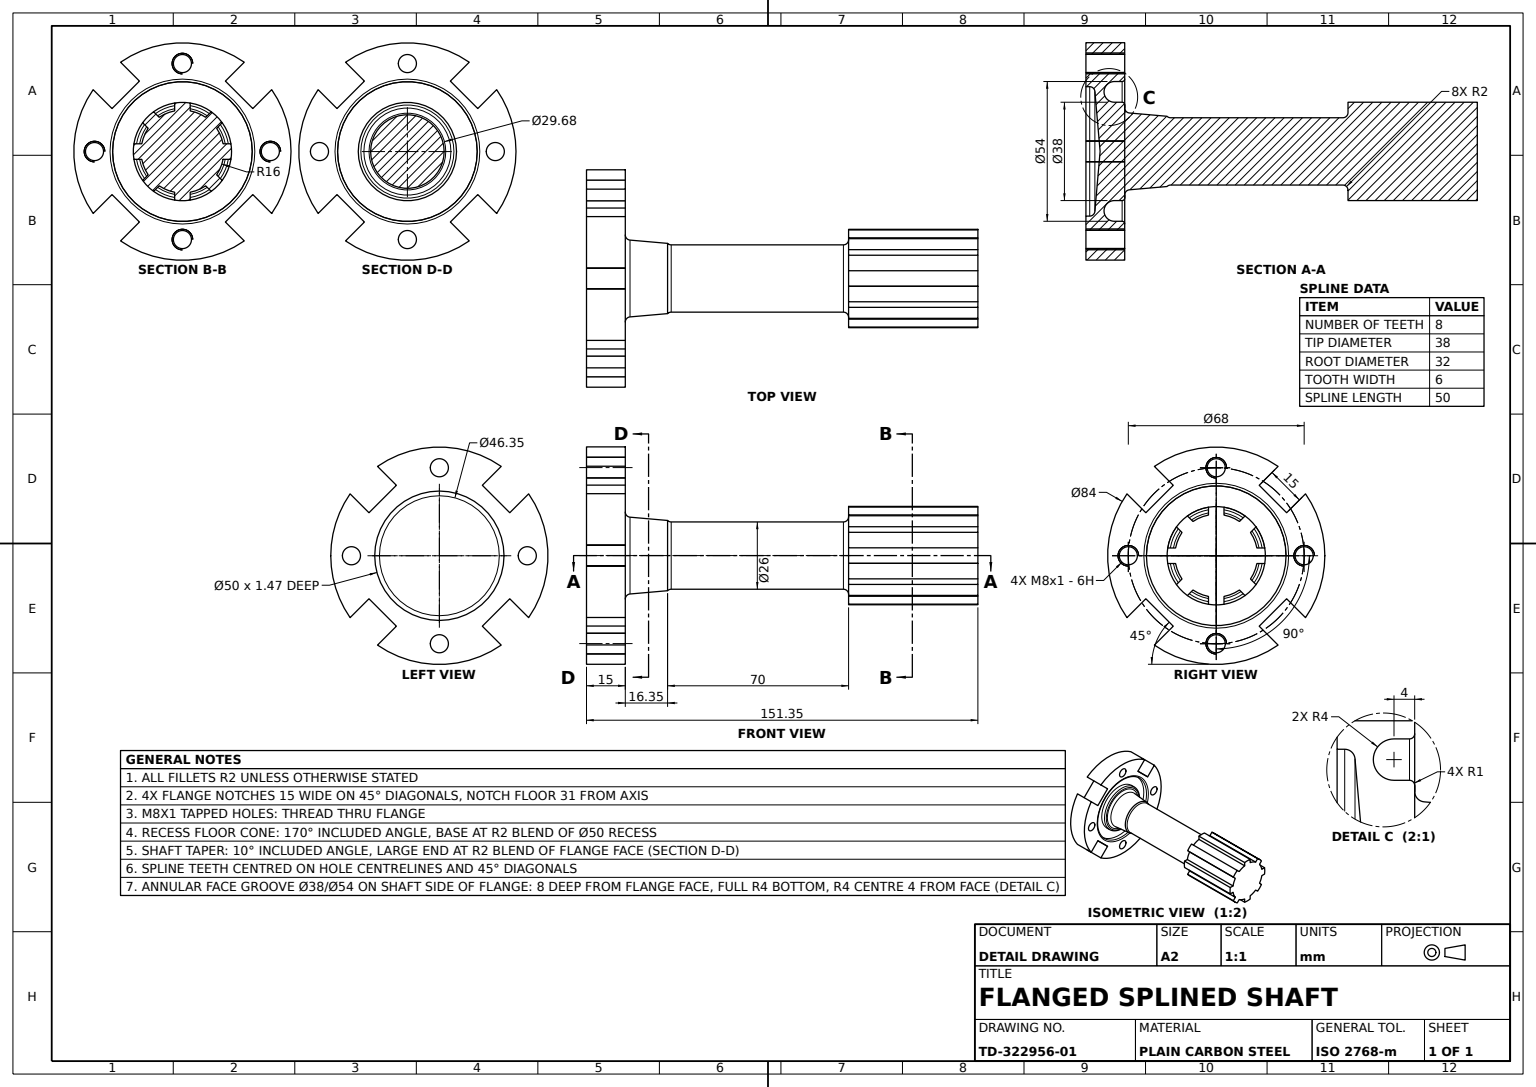
solid
v1 (0,99.353401,13)
v2 (0,32.750895,13)
e1 v1 v2 LINE
v3 (0,99.353401,-13)
e2 v1 v3 CIRCLE(AX(P(0,99.353401,0),D(0,-1,0),D(0,0,1)),13)
v4 (0,32.750895,-13)
e3 v3 v4 LINE
e4 v4 v2 CIRCLE(AX(P(0,32.750895,0),D(0,1,0),D(0,0,-1)),13)
face CYL(AX(P(0,0,0),D(0,-1,0),D(0,0,-1)),13) [-e1 e2 e3 e4]
v5 (0,1.467338,-25)
v6 (0,1.467338,25)
e5 v5 v6 CIRCLE(AX(P(0,1.467338,0),D(0,-1,0),D(0,0,-1)),25)
v7 (0,3.459727,23.174311)
e6 v7 v6 CIRCLE(AX(P(0,1.467338,23),D(1,0,0),D(0,0,-1)),2)
v8 (0,3.459727,-23.174311)
e7 v8 v7 CIRCLE(AX(P(0,3.459727,0),D(0,-1,0),D(0,0,-1)),23.174311)
e8 v8 v5 CIRCLE(AX(P(0,1.467338,-23),D(-1,0,0),D(0,0,1)),2)
face TORUS(AX(P(0,1.467338,0),D(0,-1,0),D(0,0,-1)),23,2) rev [e5 -e6 -e7 e8]
v9 (0,16.825689,14.840273)
v10 (0,16.825689,-14.840273)
e9 v9 v10 CIRCLE(AX(P(0,16.825689,0),D(0,1,0),D(0,0,-1)),14.840273)
v11 (0,15,16.832662)
e10 v9 v11 CIRCLE(AX(P(0,17,16.832662),D(-1,0,0),D(0,0,1)),2)
v12 (0,15,-16.832662)
e11 v12 v11 CIRCLE(AX(P(0,15,0),D(0,-1,0),D(0,0,1)),16.832662)
e12 v10 v12 CIRCLE(AX(P(0,17,-16.832662),D(1,0,0),D(0,0,-1)),2)
face TORUS(AX(P(0,17,0),D(0,1,0),D(0,0,1)),16.832662,2) rev [-e9 e10 -e11 -e12]
e13 v6 v5 CIRCLE(AX(P(0,1.467338,0),D(0,-1,0),D(0,0,-1)),25)
e14 v7 v8 CIRCLE(AX(P(0,3.459727,0),D(0,-1,0),D(0,0,-1)),23.174311)
face TORUS(AX(P(0,1.467338,0),D(0,-1,0),D(0,0,-1)),23,2) rev [e6 e13 -e8 -e14]
v13 (0,0,-30.5)
v14 (0,0,-37.5)
e15 v13 v14 CIRCLE(AX(P(0,0,-34),D(0,1,0),D(0,0,1)),3.5)
v15 (0,15,-30.5)
e16 v13 v15 LINE
v16 (0,15,-37.5)
e17 v15 v16 CIRCLE(AX(P(0,15,-34),D(0,1,0),D(0,0,1)),3.5)
e18 v14 v16 LINE
face CYL(AX(P(0,15,-34),D(0,1,0),D(0,0,1)),3.5) rev [-e15 e16 e17 -e18]
v17 (23.917839,15,-34.52444)
v18 (0,15,-42)
e19 v17 v18 CIRCLE(AX(P(0,15,0),D(0,1,0),D(0,0,1)),42)
v19 (23.917839,0,-34.52444)
e20 v17 v19 LINE
v20 (0,0,-42)
e21 v19 v20 CIRCLE(AX(P(0,0,0),D(0,1,0),D(0,0,1)),42)
e22 v18 v20 LINE
face CYL(AX(P(0,15,0),D(0,-1,0),D(0,0,-1)),42) [-e19 e20 e21 -e22]
v21 (0,11,27)
v22 (0,11,-27)
e23 v21 v22 CIRCLE(AX(P(0,11,0),D(0,-1,0),D(0,0,-1)),27)
v23 (0,14,-27)
e24 v23 v22 LINE
v24 (0,14,27)
e25 v23 v24 CIRCLE(AX(P(0,14,0),D(0,1,0),D(0,0,1)),27)
e26 v24 v21 LINE
face CYL(AX(P(0,0,0),D(0,-1,0),D(0,0,-1)),27) rev [e23 -e24 e25 e26]
v25 (-13.234376,151.353401,8.991735)
v26 (-13.234376,101.353401,8.991735)
e27 v25 v26 LINE
v27 (-15.716234,151.353401,3)
e28 v27 v25 CIRCLE(AX(P(0,151.353401,0),D(0,1,0),D(0,0,1)),16)
v28 (-15.716234,101.353401,3)
e29 v27 v28 LINE
e30 v28 v26 CIRCLE(AX(P(0,101.353401,0),D(0,1,0),D(0,0,1)),16)
face CYL(AX(P(0,151.353401,0),D(0,-1,0),D(0,0,-1)),16) [-e27 -e28 e29 e30]
v29 (0,0,25)
e31 v6 v29 LINE
v30 (0,0,-25)
e32 v5 v30 LINE
e33 v30 v29 CIRCLE(AX(P(0,0,0),D(0,-1,0),D(0,0,-1)),25)
face CYL(AX(P(0,0,0),D(0,-1,0),D(0,0,-1)),25) rev [-e31 -e5 e32 e33]
v31 (3,151.353401,-18.761663)
v32 (3,101.353401,-18.761663)
e34 v31 v32 LINE
v33 (3,151.353401,-15.716234)
e35 v33 v31 LINE
v34 (3,101.353401,-15.716234)
e36 v33 v34 LINE
e37 v34 v32 LINE
face PLANE(AX(P(3,151.353401,-15.716234),D(-1,0,0),D(0,0,1))) rev [-e34 -e35 e36 e37]
v35 (27.223611,15,16.617009)
v36 (27.223611,0,16.617009)
e38 v35 v36 LINE
v37 (34.52444,0,23.917839)
e39 v36 v37 LINE
v38 (34.52444,15,23.917839)
e40 v38 v37 LINE
e41 v35 v38 LINE
face PLANE(AX(P(34.52444,15,23.917839),D(0.707106781,0,-0.707106781),D(-0.707106781,0,-0.707106781))) rev [e38 e39 -e40 -e41]
v39 (0,31.353401,-13.569263)
e42 v39 v10 LINE
v40 (0,31.353401,13.569263)
e43 v39 v40 CIRCLE(AX(P(0,31.353401,0),D(0,-1,0),D(0,0,-1)),13.569263)
e44 v40 v9 LINE
face CONE(AX(P(0,15,0),D(0,-1,0),D(0,0,-1)),15,0.087266463) [e9 -e42 e43 e44]
v41 (-11.145179,151.353401,-15.38782)
v42 (-15.38782,151.353401,-11.145179)
e45 v41 v42 CIRCLE(AX(P(0,151.353401,0),D(0,1,0),D(0,0,1)),19)
v43 (-11.145179,101.353401,-15.38782)
e46 v41 v43 LINE
v44 (-15.38782,101.353401,-11.145179)
e47 v43 v44 CIRCLE(AX(P(0,101.353401,0),D(0,1,0),D(0,0,1)),19)
e48 v42 v44 LINE
face CYL(AX(P(0,151.353401,0),D(0,-1,0),D(0,0,-1)),19) [-e45 e46 e47 -e48]
v45 (-18.761663,151.353401,3)
v46 (-18.761663,101.353401,3)
e49 v45 v46 LINE
v47 (-18.761663,151.353401,-3)
e50 v47 v45 CIRCLE(AX(P(0,151.353401,0),D(0,1,0),D(0,0,1)),19)
v48 (-18.761663,101.353401,-3)
e51 v47 v48 LINE
e52 v48 v46 CIRCLE(AX(P(0,101.353401,0),D(0,1,0),D(0,0,1)),19)
face CYL(AX(P(0,151.353401,0),D(0,-1,0),D(0,0,-1)),19) [-e49 -e50 e51 e52]
v49 (0,15,-28)
e53 v49 v23 CIRCLE(AX(P(0,14,-28),D(1,0,0),D(0,0,-1)),1)
v50 (0,15,28)
e54 v50 v49 CIRCLE(AX(P(0,15,0),D(0,-1,0),D(0,0,1)),28)
e55 v50 v24 CIRCLE(AX(P(0,14,28),D(-1,0,0),D(0,0,1)),1)
face TORUS(AX(P(0,14,0),D(0,1,0),D(0,0,1)),28,1) [-e53 -e54 e55 -e25]
v51 (-8.991735,151.353401,-13.234376)
v52 (-8.991735,101.353401,-13.234376)
e56 v51 v52 LINE
v53 (-3,151.353401,-15.716234)
e57 v53 v51 CIRCLE(AX(P(0,151.353401,0),D(0,1,0),D(0,0,1)),16)
v54 (-3,101.353401,-15.716234)
e58 v53 v54 LINE
e59 v54 v52 CIRCLE(AX(P(0,101.353401,0),D(0,1,0),D(0,0,1)),16)
face CYL(AX(P(0,151.353401,0),D(0,-1,0),D(0,0,-1)),16) [-e56 -e57 e58 e59]
v55 (0,14,19)
v56 (0,15,18)
e60 v55 v56 CIRCLE(AX(P(0,14,18),D(-1,0,0),D(0,0,1)),1)
v57 (0,15,-18)
e61 v57 v56 CIRCLE(AX(P(0,15,0),D(0,1,0),D(0,0,1)),18)
v58 (0,14,-19)
e62 v58 v57 CIRCLE(AX(P(0,14,-18),D(1,0,0),D(0,0,-1)),1)
e63 v55 v58 CIRCLE(AX(P(0,14,0),D(0,-1,0),D(0,0,1)),19)
face TORUS(AX(P(0,14,0),D(0,1,0),D(0,0,1)),18,1) [e60 -e61 -e62 -e63]
v59 (11.145179,151.353401,-15.38782)
v60 (11.145179,101.353401,-15.38782)
e64 v59 v60 LINE
v61 (15.38782,151.353401,-11.145179)
e65 v61 v59 CIRCLE(AX(P(0,151.353401,0),D(0,1,0),D(0,0,1)),19)
v62 (15.38782,101.353401,-11.145179)
e66 v61 v62 LINE
e67 v62 v60 CIRCLE(AX(P(0,101.353401,0),D(0,1,0),D(0,0,1)),19)
face CYL(AX(P(0,151.353401,0),D(0,-1,0),D(0,0,-1)),19) [-e64 -e65 e66 e67]
v63 (0,0,37.5)
v64 (0,15,37.5)
e68 v63 v64 LINE
v65 (0,15,30.5)
e69 v64 v65 CIRCLE(AX(P(0,15,34),D(0,1,0),D(0,0,1)),3.5)
v66 (0,0,30.5)
e70 v66 v65 LINE
e71 v63 v66 CIRCLE(AX(P(0,0,34),D(0,1,0),D(0,0,1)),3.5)
face CYL(AX(P(0,15,34),D(0,1,0),D(0,0,1)),3.5) rev [e68 e69 -e70 -e71]
e72 v11 v12 CIRCLE(AX(P(0,15,0),D(0,-1,0),D(0,0,1)),16.832662)
e73 v56 v57 CIRCLE(AX(P(0,15,0),D(0,1,0),D(0,0,1)),18)
face PLANE(AX(P(0,15,0),D(0,1,0),D(0,0,1))) [e72 e11] [e73 e61]
v67 (-34,15,3.5)
v68 (-34,15,-3.5)
e74 v67 v68 CIRCLE(AX(P(-34,15,0),D(0,1,0),D(0,0,1)),3.5)
v69 (-34,0,-3.5)
e75 v69 v68 LINE
v70 (-34,0,3.5)
e76 v70 v69 CIRCLE(AX(P(-34,0,0),D(0,1,0),D(0,0,1)),3.5)
e77 v70 v67 LINE
face CYL(AX(P(-34,15,0),D(0,1,0),D(0,0,1)),3.5) rev [e74 -e75 -e76 e77]
v71 (-3,151.353401,-18.761663)
e78 v71 v53 LINE
e79 v51 v41 LINE
v72 (-13.234376,151.353401,-8.991735)
e80 v42 v72 LINE
v73 (-15.716234,151.353401,-3)
e81 v72 v73 CIRCLE(AX(P(0,151.353401,0),D(0,1,0),D(0,0,1)),16)
e82 v73 v47 LINE
e83 v45 v27 LINE
v74 (-15.38782,151.353401,11.145179)
e84 v25 v74 LINE
v75 (-11.145179,151.353401,15.38782)
e85 v74 v75 CIRCLE(AX(P(0,151.353401,0),D(0,1,0),D(0,0,1)),19)
v76 (-8.991735,151.353401,13.234376)
e86 v75 v76 LINE
v77 (-3,151.353401,15.716234)
e87 v76 v77 CIRCLE(AX(P(0,151.353401,0),D(0,1,0),D(0,0,1)),16)
v78 (-3,151.353401,18.761663)
e88 v77 v78 LINE
v79 (3,151.353401,18.761663)
e89 v78 v79 CIRCLE(AX(P(0,151.353401,0),D(0,1,0),D(0,0,1)),19)
v80 (3,151.353401,15.716234)
e90 v79 v80 LINE
v81 (8.991735,151.353401,13.234376)
e91 v80 v81 CIRCLE(AX(P(0,151.353401,0),D(0,1,0),D(0,0,1)),16)
v82 (11.145179,151.353401,15.38782)
e92 v81 v82 LINE
v83 (15.38782,151.353401,11.145179)
e93 v82 v83 CIRCLE(AX(P(0,151.353401,0),D(0,1,0),D(0,0,1)),19)
v84 (13.234376,151.353401,8.991735)
e94 v83 v84 LINE
v85 (15.716234,151.353401,3)
e95 v84 v85 CIRCLE(AX(P(0,151.353401,0),D(0,1,0),D(0,0,1)),16)
v86 (18.761663,151.353401,3)
e96 v85 v86 LINE
v87 (18.761663,151.353401,-3)
e97 v86 v87 CIRCLE(AX(P(0,151.353401,0),D(0,1,0),D(0,0,1)),19)
v88 (15.716234,151.353401,-3)
e98 v87 v88 LINE
v89 (13.234376,151.353401,-8.991735)
e99 v88 v89 CIRCLE(AX(P(0,151.353401,0),D(0,1,0),D(0,0,1)),16)
e100 v89 v61 LINE
v90 (8.991735,151.353401,-13.234376)
e101 v59 v90 LINE
e102 v90 v33 CIRCLE(AX(P(0,151.353401,0),D(0,1,0),D(0,0,1)),16)
v91 (0,151.353401,-19)
e103 v31 v91 CIRCLE(AX(P(0,151.353401,0),D(0,1,0),D(0,0,1)),19)
e104 v91 v71 CIRCLE(AX(P(0,151.353401,0),D(0,1,0),D(0,0,1)),19)
face PLANE(AX(P(0,151.353401,0),D(0,1,0),D(0,0,1))) [e78 e57 e79 e45 e80 e81 e82 e50 e83 e28 e84 e85 e86 e87 e88 e89 e90 e91 e92 e93 e94 e95 e96 e97 e98 e99 e100 e65 e101 e102 e35 e103 e104]
v92 (-23.917839,15,34.52444)
v93 (23.917839,15,34.52444)
e105 v92 v93 CIRCLE(AX(P(0,15,0),D(0,1,0),D(0,0,1)),42)
v94 (-23.917839,0,34.52444)
e106 v92 v94 LINE
v95 (23.917839,0,34.52444)
e107 v94 v95 CIRCLE(AX(P(0,0,0),D(0,1,0),D(0,0,1)),42)
e108 v93 v95 LINE
face CYL(AX(P(0,15,0),D(0,-1,0),D(0,0,-1)),42) [-e105 e106 e107 -e108]
v96 (-3,101.353401,15.716234)
e109 v77 v96 LINE
v97 (-3,101.353401,18.761663)
e110 v96 v97 LINE
e111 v78 v97 LINE
face PLANE(AX(P(-3,151.353401,15.716234),D(1,0,0),D(0,0,-1))) rev [e109 e110 -e111 -e88]
v98 (8.991735,101.353401,-13.234376)
e112 v90 v98 LINE
e113 v98 v34 CIRCLE(AX(P(0,101.353401,0),D(0,1,0),D(0,0,1)),16)
face CYL(AX(P(0,151.353401,0),D(0,-1,0),D(0,0,-1)),16) [-e102 e112 e113 -e36]
v99 (0,5.487217,0)
e114 v99 v7 LINE
e115 v99 v8 LINE
face CONE(AX(P(0,3.459727,0),D(0,-1,0),D(0,0,-1)),23.174311485,1.483529864) rev [-e114 e115 e7]
e116 v2 v4 CIRCLE(AX(P(0,32.750895,0),D(0,1,0),D(0,0,-1)),13)
e117 v3 v1 CIRCLE(AX(P(0,99.353401,0),D(0,-1,0),D(0,0,1)),13)
face CYL(AX(P(0,0,0),D(0,-1,0),D(0,0,-1)),13) [e1 e116 -e3 e117]
v100 (15.38782,101.353401,11.145179)
v101 (13.234376,101.353401,8.991735)
e118 v100 v101 LINE
e119 v84 v101 LINE
e120 v83 v100 LINE
face PLANE(AX(P(13.234376,151.353401,8.991735),D(-0.707106781,0,0.707106781),D(0.707106781,0,0.707106781))) rev [e118 -e119 -e94 e120]
v102 (-16.617009,15,27.223611)
e121 v102 v92 LINE
v103 (-16.617009,0,27.223611)
e122 v102 v103 LINE
e123 v103 v94 LINE
face PLANE(AX(P(-23.917839,15,34.52444),D(0.707106781,0,0.707106781),D(0.707106781,0,-0.707106781))) rev [-e121 e122 e123 -e106]
v104 (-34.52444,15,-23.917839)
v105 (-34.52444,15,23.917839)
e124 v104 v105 CIRCLE(AX(P(0,15,0),D(0,1,0),D(0,0,1)),42)
v106 (-34.52444,0,-23.917839)
e125 v104 v106 LINE
v107 (-34.52444,0,23.917839)
e126 v106 v107 CIRCLE(AX(P(0,0,0),D(0,1,0),D(0,0,1)),42)
e127 v105 v107 LINE
face CYL(AX(P(0,15,0),D(0,-1,0),D(0,0,-1)),42) [-e124 e125 e126 -e127]
e128 v52 v43 LINE
face PLANE(AX(P(-8.991735,151.353401,-13.234376),D(-0.707106781,0,0.707106781),D(0.707106781,0,0.707106781))) rev [e128 -e46 -e79 e56]
v108 (0,11,-19)
e129 v22 v108 CIRCLE(AX(P(0,11,-23),D(-1,0,0),D(0,0,1)),4)
v109 (0,11,19)
e130 v21 v109 CIRCLE(AX(P(0,11,23),D(1,0,0),D(0,0,-1)),4)
e131 v109 v108 CIRCLE(AX(P(0,11,0),D(0,-1,0),D(0,0,-1)),19)
face TORUS(AX(P(0,11,0),D(0,-1,0),D(0,0,-1)),23,4) rev [-e129 -e23 e130 e131]
v110 (-3,101.353401,-18.761663)
e132 v110 v54 LINE
e133 v71 v110 LINE
face PLANE(AX(P(-3,151.353401,-15.716234),D(1,0,0),D(0,0,-1))) rev [e132 -e58 -e78 e133]
v111 (0,101.353401,15)
e134 v111 v1 CIRCLE(AX(P(0,99.353401,15),D(-1,0,0),D(0,0,1)),2)
v112 (0,101.353401,-15)
e135 v112 v111 CIRCLE(AX(P(0,101.353401,0),D(0,1,0),D(0,0,1)),15)
e136 v112 v3 CIRCLE(AX(P(0,99.353401,-15),D(1,0,0),D(0,0,-1)),2)
face TORUS(AX(P(0,99.353401,0),D(0,1,0),D(0,0,1)),15,2) rev [-e2 -e134 -e135 e136]
v113 (8.991735,101.353401,13.234376)
e137 v81 v113 LINE
v114 (3,101.353401,15.716234)
e138 v80 v114 LINE
e139 v114 v113 CIRCLE(AX(P(0,101.353401,0),D(0,1,0),D(0,0,1)),16)
face CYL(AX(P(0,151.353401,0),D(0,-1,0),D(0,0,-1)),16) [-e137 -e91 e138 e139]
v115 (-27.223611,15,16.617009)
e140 v115 v102 LINE
v116 (-27.223611,0,16.617009)
e141 v115 v116 LINE
e142 v116 v103 LINE
face PLANE(AX(P(-16.617009,15,27.223611),D(0.707106781,0,-0.707106781),D(-0.707106781,0,-0.707106781))) rev [-e140 e141 e142 -e122]
v117 (3,101.353401,18.761663)
e143 v117 v114 LINE
e144 v97 v117 CIRCLE(AX(P(0,101.353401,0),D(0,1,0),D(0,0,1)),19)
v118 (-8.991735,101.353401,13.234376)
e145 v118 v96 CIRCLE(AX(P(0,101.353401,0),D(0,1,0),D(0,0,1)),16)
v119 (-11.145179,101.353401,15.38782)
e146 v119 v118 LINE
v120 (-15.38782,101.353401,11.145179)
e147 v120 v119 CIRCLE(AX(P(0,101.353401,0),D(0,1,0),D(0,0,1)),19)
e148 v26 v120 LINE
e149 v46 v28 LINE
v121 (-15.716234,101.353401,-3)
e150 v121 v48 LINE
v122 (-13.234376,101.353401,-8.991735)
e151 v122 v121 CIRCLE(AX(P(0,101.353401,0),D(0,1,0),D(0,0,1)),16)
e152 v44 v122 LINE
v123 (0,101.353401,-19)
e153 v123 v110 CIRCLE(AX(P(0,101.353401,0),D(0,1,0),D(0,0,1)),19)
e154 v32 v123 CIRCLE(AX(P(0,101.353401,0),D(0,1,0),D(0,0,1)),19)
e155 v60 v98 LINE
v124 (13.234376,101.353401,-8.991735)
e156 v124 v62 LINE
v125 (15.716234,101.353401,-3)
e157 v125 v124 CIRCLE(AX(P(0,101.353401,0),D(0,1,0),D(0,0,1)),16)
v126 (18.761663,101.353401,-3)
e158 v126 v125 LINE
v127 (18.761663,101.353401,3)
e159 v127 v126 CIRCLE(AX(P(0,101.353401,0),D(0,1,0),D(0,0,1)),19)
v128 (15.716234,101.353401,3)
e160 v128 v127 LINE
e161 v101 v128 CIRCLE(AX(P(0,101.353401,0),D(0,1,0),D(0,0,1)),16)
v129 (11.145179,101.353401,15.38782)
e162 v129 v100 CIRCLE(AX(P(0,101.353401,0),D(0,1,0),D(0,0,1)),19)
e163 v113 v129 LINE
e164 v111 v112 CIRCLE(AX(P(0,101.353401,0),D(0,1,0),D(0,0,1)),15)
face PLANE(AX(P(0,101.353401,0),D(0,1,0),D(0,0,1))) rev [-e139 -e143 -e144 -e110 -e145 -e146 -e147 -e148 -e30 -e149 -e52 -e150 -e151 -e152 -e47 -e128 -e59 -e132 -e153 -e154 -e37 -e113 -e155 -e67 -e156 -e157 -e158 -e159 -e160 -e161 -e118 -e162 -e163] [e164 e135]
v130 (34.52444,0,-23.917839)
v131 (27.223611,0,-16.617009)
e165 v130 v131 LINE
v132 (27.223611,15,-16.617009)
e166 v132 v131 LINE
v133 (34.52444,15,-23.917839)
e167 v133 v132 LINE
e168 v133 v130 LINE
face PLANE(AX(P(27.223611,15,-16.617009),D(0.707106781,0,0.707106781),D(0.707106781,0,-0.707106781))) rev [e165 -e166 -e167 e168]
v134 (34,15,3.5)
v135 (34,15,-3.5)
e169 v134 v135 CIRCLE(AX(P(34,15,0),D(0,1,0),D(0,0,1)),3.5)
v136 (34,0,-3.5)
e170 v136 v135 LINE
v137 (34,0,3.5)
e171 v137 v136 CIRCLE(AX(P(34,0,0),D(0,1,0),D(0,0,1)),3.5)
e172 v137 v134 LINE
face CYL(AX(P(34,15,0),D(0,1,0),D(0,0,1)),3.5) rev [e169 -e170 -e171 e172]
e173 v37 v130 CIRCLE(AX(P(0,0,0),D(0,1,0),D(0,0,1)),42)
e174 v38 v133 CIRCLE(AX(P(0,15,0),D(0,1,0),D(0,0,1)),42)
face CYL(AX(P(0,15,0),D(0,-1,0),D(0,0,-1)),42) [e173 -e168 -e174 e40]
e175 v105 v115 LINE
e176 v107 v116 LINE
face PLANE(AX(P(-27.223611,15,16.617009),D(-0.707106781,0,-0.707106781),D(-0.707106781,0,0.707106781))) rev [-e141 -e175 e127 e176]
e177 v86 v127 LINE
e178 v85 v128 LINE
face PLANE(AX(P(15.716234,151.353401,3),D(0,0,-1),D(-1,0,0))) rev [e160 -e177 -e96 e178]
v138 (16.617009,15,27.223611)
v139 (16.617009,0,27.223611)
e179 v138 v139 LINE
e180 v139 v36 LINE
e181 v138 v35 LINE
face PLANE(AX(P(27.223611,15,16.617009),D(-0.707106781,0,-0.707106781),D(-0.707106781,0,0.707106781))) rev [e179 e180 -e38 -e181]
v140 (-23.917839,0,-34.52444)
e182 v20 v140 CIRCLE(AX(P(0,0,0),D(0,1,0),D(0,0,1)),42)
v141 (-23.917839,15,-34.52444)
e183 v141 v140 LINE
e184 v18 v141 CIRCLE(AX(P(0,15,0),D(0,1,0),D(0,0,1)),42)
face CYL(AX(P(0,15,0),D(0,-1,0),D(0,0,-1)),42) [e182 -e183 -e184 e22]
e185 v10 v9 CIRCLE(AX(P(0,16.825689,0),D(0,1,0),D(0,0,-1)),14.840273)
e186 v40 v39 CIRCLE(AX(P(0,31.353401,0),D(0,-1,0),D(0,0,-1)),13.569263)
face CONE(AX(P(0,15,0),D(0,-1,0),D(0,0,-1)),15,0.087266463) [e185 -e44 e186 e42]
face TORUS(AX(P(0,17,0),D(0,1,0),D(0,0,1)),16.832662,2) rev [e12 -e72 -e10 -e185]
v142 (-16.617009,15,-27.223611)
e187 v141 v142 LINE
v143 (-16.617009,0,-27.223611)
e188 v140 v143 LINE
e189 v142 v143 LINE
face PLANE(AX(P(-16.617009,15,-27.223611),D(0.707106781,0,-0.707106781),D(-0.707106781,0,-0.707106781))) rev [-e187 e183 e188 -e189]
e190 v58 v108 LINE
e191 v58 v55 CIRCLE(AX(P(0,14,0),D(0,-1,0),D(0,0,1)),19)
e192 v55 v109 LINE
e193 v108 v109 CIRCLE(AX(P(0,11,0),D(0,-1,0),D(0,0,-1)),19)
face CYL(AX(P(0,0,0),D(0,-1,0),D(0,0,-1)),19) [-e190 e191 e192 -e193]
e194 v89 v124 LINE
face PLANE(AX(P(13.234376,151.353401,-8.991735),D(-0.707106781,0,-0.707106781),D(-0.707106781,0,0.707106781))) rev [-e100 e194 e156 -e66]
e195 v75 v119 LINE
e196 v76 v118 LINE
face PLANE(AX(P(-8.991735,151.353401,13.234376),D(-0.707106781,0,-0.707106781),D(-0.707106781,0,0.707106781))) rev [e195 e146 -e196 -e86]
face CYL(AX(P(0,151.353401,0),D(0,-1,0),D(0,0,-1)),16) [e119 e161 -e178 -e95]
e197 v69 v70 CIRCLE(AX(P(-34,0,0),D(0,1,0),D(0,0,1)),3.5)
e198 v68 v67 CIRCLE(AX(P(-34,15,0),D(0,1,0),D(0,0,1)),3.5)
face CYL(AX(P(-34,15,0),D(0,1,0),D(0,0,1)),3.5) rev [-e77 -e197 e75 e198]
face TORUS(AX(P(0,99.353401,0),D(0,1,0),D(0,0,1)),15,2) rev [-e164 e134 -e117 -e136]
v144 (-27.223611,0,-16.617009)
e199 v144 v106 LINE
e200 v143 v144 LINE
v145 (16.617009,0,-27.223611)
e201 v145 v19 LINE
e202 v131 v145 LINE
e203 v95 v139 LINE
e204 v14 v13 CIRCLE(AX(P(0,0,-34),D(0,1,0),D(0,0,1)),3.5)
e205 v29 v30 CIRCLE(AX(P(0,0,0),D(0,-1,0),D(0,0,-1)),25)
e206 v136 v137 CIRCLE(AX(P(34,0,0),D(0,1,0),D(0,0,1)),3.5)
e207 v66 v63 CIRCLE(AX(P(0,0,34),D(0,1,0),D(0,0,1)),3.5)
face PLANE(AX(P(0,0,0),D(0,1,0),D(0,0,1))) rev [e197 e76] [-e142 -e176 -e126 -e199 -e200 -e188 -e182 -e21 -e201 -e202 -e165 -e173 -e39 -e180 -e203 -e107 -e123] [e204 e15] [-e33 -e205] [e206 e171] [e207 e71]
e208 v74 v120 LINE
face PLANE(AX(P(-13.234376,151.353401,8.991735),D(0.707106781,0,0.707106781),D(0.707106781,0,-0.707106781))) rev [-e84 e27 e148 -e208]
face CYL(AX(P(0,151.353401,0),D(0,-1,0),D(0,0,-1)),19) [e208 e147 -e195 -e85]
e209 v16 v15 CIRCLE(AX(P(0,15,-34),D(0,1,0),D(0,0,1)),3.5)
face CYL(AX(P(0,15,-34),D(0,1,0),D(0,0,1)),3.5) rev [-e204 e18 e209 -e16]
face CYL(AX(P(0,151.353401,0),D(0,-1,0),D(0,0,-1)),16) [e145 -e109 -e87 e196]
e210 v73 v121 LINE
e211 v72 v122 LINE
face CYL(AX(P(0,151.353401,0),D(0,-1,0),D(0,0,-1)),16) [e151 -e210 -e81 e211]
face PLANE(AX(P(-13.234376,151.353401,-8.991735),D(0.707106781,0,-0.707106781),D(-0.707106781,0,-0.707106781))) rev [-e211 -e80 e48 e152]
face CYL(AX(P(0,0,0),D(0,-1,0),D(0,0,-1)),25) rev [-e32 -e13 e31 e205]
e212 v22 v21 CIRCLE(AX(P(0,11,0),D(0,-1,0),D(0,0,-1)),27)
e213 v24 v23 CIRCLE(AX(P(0,14,0),D(0,1,0),D(0,0,1)),27)
face CYL(AX(P(0,0,0),D(0,-1,0),D(0,0,-1)),27) rev [e24 e212 -e26 e213]
e214 v87 v126 LINE
face CYL(AX(P(0,151.353401,0),D(0,-1,0),D(0,0,-1)),19) [-e214 -e97 e177 e159]
e215 v39 v4 CIRCLE(AX(P(0,32.750895,-15),D(-1,0,0),D(0,0,1)),2)
e216 v40 v2 CIRCLE(AX(P(0,32.750895,15),D(1,0,0),D(0,0,-1)),2)
face TORUS(AX(P(0,32.750895,0),D(0,-1,0),D(0,0,-1)),15,2) rev [-e215 -e186 e216 -e4]
face CONE(AX(P(0,3.459727,0),D(0,-1,0),D(0,0,-1)),23.174311485,1.483529864) rev [e14 -e115 e114]
e217 v88 v125 LINE
face PLANE(AX(P(15.716234,151.353401,-3),D(0,0,1),D(1,0,0))) rev [e158 -e217 -e98 e214]
e218 v82 v129 LINE
face PLANE(AX(P(8.991735,151.353401,13.234376),D(0.707106781,0,-0.707106781),D(-0.707106781,0,-0.707106781))) rev [-e218 -e92 e137 e163]
face CYL(AX(P(0,151.353401,0),D(0,-1,0),D(0,0,-1)),19) [-e93 e218 e162 -e120]
e219 v135 v134 CIRCLE(AX(P(34,15,0),D(0,1,0),D(0,0,1)),3.5)
face CYL(AX(P(34,15,0),D(0,1,0),D(0,0,1)),3.5) rev [-e206 e170 e219 -e172]
face PLANE(AX(P(-15.716234,151.353401,3),D(0,0,-1),D(-1,0,0))) rev [-e83 e49 e149 -e29]
face TORUS(AX(P(0,11,0),D(0,-1,0),D(0,0,-1)),23,4) rev [e193 -e130 -e212 e129]
face CYL(AX(P(0,0,0),D(0,-1,0),D(0,0,-1)),19) [e63 e190 -e131 -e192]
face PLANE(AX(P(8.991735,151.353401,-13.234376),D(0.707106781,0,0.707106781),D(0.707106781,0,-0.707106781))) rev [e64 e155 -e112 -e101]
v146 (16.617009,15,-27.223611)
e220 v132 v146 LINE
e221 v146 v17 LINE
v147 (-27.223611,15,-16.617009)
e222 v142 v147 LINE
e223 v147 v104 LINE
e224 v93 v138 LINE
e225 v65 v64 CIRCLE(AX(P(0,15,34),D(0,1,0),D(0,0,1)),3.5)
e226 v49 v50 CIRCLE(AX(P(0,15,0),D(0,-1,0),D(0,0,1)),28)
face PLANE(AX(P(0,15,0),D(0,1,0),D(0,0,1))) [-e169 -e219] [e174 e167 e220 e221 e19 e184 e187 e222 e223 e124 e175 e140 e121 e105 e224 e181 e41] [-e225 -e69] [e54 e226] [-e17 -e209] [-e74 -e198]
face CYL(AX(P(0,15,34),D(0,1,0),D(0,0,1)),3.5) rev [-e207 e70 e225 -e68]
e227 v91 v123 LINE
face CYL(AX(P(0,151.353401,0),D(0,-1,0),D(0,0,-1)),19) [-e103 e34 e154 -e227]
e228 v79 v117 LINE
face CYL(AX(P(0,151.353401,0),D(0,-1,0),D(0,0,-1)),19) [-e89 e111 e144 -e228]
e229 v146 v145 LINE
face PLANE(AX(P(16.617009,15,-27.223611),D(-0.707106781,0,0.707106781),D(0.707106781,0,0.707106781))) rev [-e220 e166 e202 -e229]
face PLANE(AX(P(16.617009,15,27.223611),D(-0.707106781,0,0.707106781),D(0.707106781,0,0.707106781))) rev [e203 -e179 -e224 e108]
face CYL(AX(P(0,151.353401,0),D(0,-1,0),D(0,0,-1)),16) [e217 e157 -e194 -e99]
face PLANE(AX(P(23.917839,15,-34.52444),D(-0.707106781,0,-0.707106781),D(-0.707106781,0,0.707106781))) rev [e201 -e20 -e221 e229]
face TORUS(AX(P(0,32.750895,0),D(0,-1,0),D(0,0,-1)),15,2) rev [e215 -e116 -e216 -e43]
e230 v147 v144 LINE
face PLANE(AX(P(-27.223611,15,-16.617009),D(0.707106781,0,0.707106781),D(0.707106781,0,-0.707106781))) rev [-e230 -e222 e189 e200]
face CYL(AX(P(0,151.353401,0),D(0,-1,0),D(0,0,-1)),19) [e153 -e133 -e104 e227]
face PLANE(AX(P(3,151.353401,15.716234),D(-1,0,0),D(0,0,1))) rev [-e138 -e90 e228 e143]
face PLANE(AX(P(-15.716234,151.353401,-3),D(0,0,1),D(1,0,0))) rev [e210 e150 -e51 -e82]
face TORUS(AX(P(0,14,0),D(0,1,0),D(0,0,1)),28,1) [-e213 -e55 -e226 e53]
face TORUS(AX(P(0,14,0),D(0,1,0),D(0,0,1)),18,1) [-e191 e62 -e73 -e60]
face PLANE(AX(P(-34.52444,15,-23.917839),D(-0.707106781,0,0.707106781),D(0.707106781,0,0.707106781))) rev [-e125 -e223 e230 e199]
